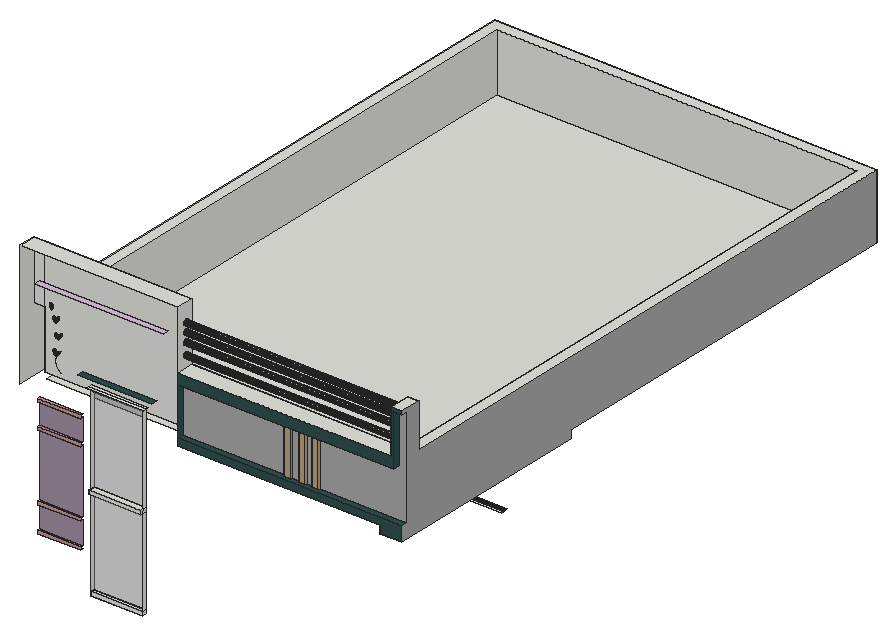
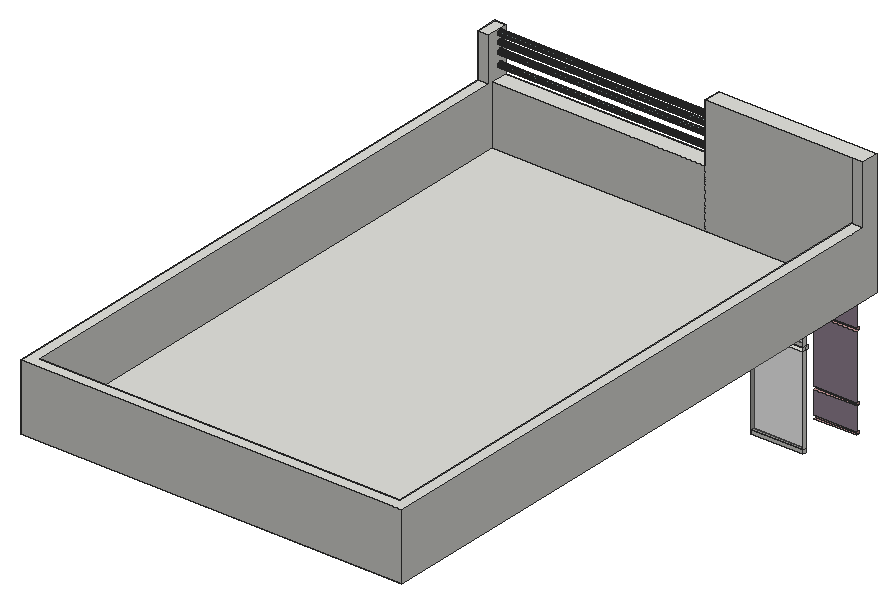
# SketchUp Ruby script. Lengths in inches.
U = 1.inch
M = Sketchup.active_model
def pt(a) = Geom::Point3d.new(a.map { |v| v * U })
def face(e, loops, mat)
  f = e.add_face(loops[0].map { |a| pt(a) })
  loops[1..].each { |l| e.add_face(l.map { |a| pt(a) }).erase! }
  f.material = f.back_material = mat if mat
  f
end
# faces: each face lists its corners as indices into pts; further lists are holes
def faces(e, pts, list, mat = nil) = list.each { |f| face(e, (f[0].is_a?(Array) ? f : [f]).map { |l| l.map { |i| pts[i] } }, mat) }
# xy, xz, yz: faces in a plane at the given z, y or x. An outline is a flat list of corners, or four numbers for a rectangle; further outlines are holes
def ring(l) = l.size == 4 ? [[l[0], l[1]], [l[2], l[1]], [l[2], l[3]], [l[0], l[3]]] : l.each_slice(2).to_a
def flat(e, list, mat, &to3) = list.each { |f| face(e, (f[0].is_a?(Array) ? f : [f]).map { |l| ring(l).map { |u, v| to3.(u, v) } }, mat) }
def xy(e, z, list, mat = nil) = flat(e, list, mat) { |x, y| [x, y, z] }
def xz(e, y, list, mat = nil) = flat(e, list, mat) { |x, z| [x, y, z] }
def yz(e, x, list, mat = nil) = flat(e, list, mat) { |y, z| [x, y, z] }
def lines(e, pts, list) = list.each { |a, b| e.add_line(pt(pts[a]), pt(pts[b])) }
# prism: a flat outline (further loops are holes) pulled along v
def prism(e, loops, v, mat = nil)
  f = face(e, loops, mat); d = Geom::Vector3d.new(v.map { |x| x * U })
  f.pushpull(f.normal.samedirection?(d) ? d.length : -d.length)
end
def box(e, o, s, mat = nil) = prism(e, [[o, [o[0] + s[0], o[1], o[2]], [o[0] + s[0], o[1] + s[1], o[2]], [o[0], o[1] + s[1], o[2]]]], [0, 0, s[2]], mat)
def at(x, y, z, deg = 0) = Geom::Transformation.translation(pt([x, y, z])) * Geom::Transformation.rotation(ORIGIN, Z_AXIS, deg.degrees)
def axes(o, x, y, z) = Geom::Transformation.new([*x, 0, *y, 0, *z, 0, *pt(o).to_a, 1])
def part(name) = M.definitions.add(name)
# library, detail: a bought-in or finely detailed component or shape, given as its bounding box
def library(name, o, s) = part(name).tap { |d| box(d.entities, o, s) }
def detail(e, o, s) = box(e.add_group.entities, o, s)
def put(e, d, t, mat = nil) = e.add_instance(d, t).tap { |i| i.material = mat if mat }
def group(e, t, mat = nil) = e.add_group.tap { |g| g.transformation = t; g.material = mat if mat }.entities
root = M.entities
M.materials.add("[0033_NavajoWhite]").color = [186, 162, 126]
M.materials.add("[0078_DarkSlateGray]").color = [47, 79, 79]
M.materials.add("[0090_LightCyan]").color = [165, 188, 188]
M.materials.add("[0118_Thistle]").color = [160, 142, 160]
M.materials.add("[0118_Thistle]1").color = [216, 191, 216]
M.materials.add("[0119_RosyBrown]").color = [198, 151, 151]
M.materials.add("[0124_Purple]").color = [128, 0, 128]
M.materials.add("[0132_LightGray]").color = [169, 169, 169]
M.materials.add("[0136_Charcoal]").color = [35, 35, 35]
M.materials.add("[Translucent Glass Gray]").color = [128, 128, 128]
M.materials["[Translucent Glass Gray]"].alpha = 0.5
xy(root,362.14,[[104.07,77,146.63,80]])
xy(root,365.14,[[104.07,77,146.63,80]])
xy(root,391.54,[[60,78,94.88,80]],"[0119_RosyBrown]")
xy(root,394.13,[[60,78,94.88,80]],"[0119_RosyBrown]")
xy(root,412.82,[[60,78,94.88,80]],"[0119_RosyBrown]")
xy(root,415.1875,[[60,78,94.88,80]],"[0119_RosyBrown]")
xy(root,418.73,[[210.99,246,254.89,248],[260.89,246,304.8,248]])
xy(root,421.73,[[257.89,248,259.89,250]])
xy(root,421.73,[[207.99,246,257.89,248],[257.89,246,259.89,248],[259.89,246,307.8,248]],"[0136_Charcoal]")
xy(root,437.14,[[104.07,75,146.63,80]])
xy(root,440.14,[[104.07,75,146.63,80]])
xy(root,467.57,[[60,78,94.88,80]],"[0119_RosyBrown]")
xy(root,469.9375,[[60,78,94.88,80]],"[0119_RosyBrown]")
xy(root,488.13,[[60,78,94.88,80]],"[0119_RosyBrown]")
xy(root,490.5,[[60,78,94.88,80]],"[0119_RosyBrown]")
xy(root,492,[[342,75,360,248]],"[0078_DarkSlateGray]")
xy(root,498,[[[177,75,177,91,57,91,57,248,342,248,342,75],[209.97,142.3125,210.74,142.46,211.45,142.79,212.04,143.3,212.49,143.95,212.75,144.68,212.8125,145.46,212.67,146.23,212.33,146.94,211.82,147.54,211.18,147.98,210.44,148.24,209.66,148.3,208.89,148.16,208.18,147.83,207.59,147.32,207.14,146.67,206.88,145.93,206.82,145.15,206.96,144.38,207.3,143.68,207.81,143.08,208.45,142.64,209.19,142.375],[279.78,204.125,280.55,204.27,281.26,204.6,281.86,205.11,282.3,205.76,282.5625,206.5,282.625,207.28,282.48,208.05,282.14,208.75,281.64,209.35,280.99,209.79,280.25,210.06,279.47,210.12,278.7,209.97,277.99,209.64,277.4,209.13,276.95,208.48,276.69,207.75,276.63,206.96,276.77,206.19,277.11,205.49,277.62,204.89,278.26,204.45,279,204.1875],[279.78,142.3125,280.55,142.46,281.26,142.79,281.86,143.3,282.3,143.95,282.5625,144.68,282.625,145.46,282.48,146.23,282.14,146.94,281.64,147.54,280.99,147.98,280.25,148.24,279.47,148.3,278.7,148.16,277.99,147.83,277.4,147.32,276.95,146.67,276.69,145.93,276.63,145.15,276.77,144.38,277.11,143.68,277.62,143.08,278.26,142.64,279,142.375],[209.97,203.6875,210.74,203.83,211.45,204.17,212.04,204.68,212.49,205.32,212.75,206.06,212.8125,206.84,212.67,207.61,212.33,208.32,211.82,208.91,211.18,209.36,210.44,209.62,209.66,209.68,208.89,209.54,208.18,209.2,207.59,208.69,207.14,208.05,206.88,207.31,206.82,206.53,206.96,205.76,207.3,205.05,207.81,204.45,208.45,204.01,209.19,203.75]],[209.97,142.3125,209.19,142.375,208.45,142.64,207.81,143.08,207.3,143.68,206.96,144.38,206.82,145.15,206.88,145.93,207.14,146.67,207.59,147.32,208.18,147.83,208.89,148.16,209.66,148.3,210.44,148.24,211.18,147.98,211.82,147.54,212.33,146.94,212.67,146.23,212.8125,145.46,212.75,144.68,212.49,143.95,212.04,143.3,211.45,142.79,210.74,142.46],[279.78,142.3125,279,142.375,278.26,142.64,277.62,143.08,277.11,143.68,276.77,144.38,276.63,145.15,276.69,145.93,276.95,146.67,277.4,147.32,277.99,147.83,278.7,148.16,279.47,148.3,280.25,148.24,280.99,147.98,281.64,147.54,282.14,146.94,282.48,146.23,282.625,145.46,282.5625,144.68,282.3,143.95,281.86,143.3,281.26,142.79,280.55,142.46],[209.97,203.6875,209.19,203.75,208.45,204.01,207.81,204.45,207.3,205.05,206.96,205.76,206.82,206.53,206.88,207.31,207.14,208.05,207.59,208.69,208.18,209.2,208.89,209.54,209.66,209.68,210.44,209.62,211.18,209.36,211.82,208.91,212.33,208.32,212.67,207.61,212.8125,206.84,212.75,206.06,212.49,205.32,212.04,204.68,211.45,204.17,210.74,203.83],[279.78,204.125,279,204.1875,278.26,204.45,277.62,204.89,277.11,205.49,276.77,206.19,276.63,206.96,276.69,207.75,276.95,208.48,277.4,209.13,277.99,209.64,278.7,209.97,279.47,210.12,280.25,210.06,280.99,209.79,281.64,209.35,282.14,208.75,282.48,208.05,282.625,207.28,282.5625,206.5,282.3,205.76,281.86,205.11,281.26,204.6,280.55,204.27],
  [[48,248,360,560],[186,257,351,551],[57,257,177,551]]])
xy(root,504,[[57,89,351,551]])
xy(root,504,[[177,75,360,75,360,80,288.56,80,288.56,78.5,283.23,78.5,283.23,80,278.12,80,278.12,78.5,272.79,78.5,272.79,80,266.31,80,266.31,78.5,260.98,78.5,260.98,80,177,80]],"[0078_DarkSlateGray]")
xy(root,512.14,[[104.07,77,146.63,80]])
xy(root,514.14,[[102.07,75,148.63,77],[102.07,77,148.63,80]])
xy(root,521.33,[[94.88,75,155.82,80]],"[0078_DarkSlateGray]")
xy(root,543,[[177,75,177,80,260.98,80,260.98,78.5,266.31,78.5,266.31,80,272.79,80,272.79,78.5,278.12,78.5,278.12,80,283.23,80,283.23,78.5,288.56,78.5,288.56,80,353.5,80,353.5,75]],"[0078_DarkSlateGray]")
xy(root,552,[[177,75,351,89],[48,89,57,89,57,551,351,551,351,92,360,92,360,560,48,560]])
xy(root,576,[[60,75,165,80]],"[0118_Thistle]1")
xy(root,585,[[353.5,75,360,80]])
xy(root,588,[[351,75,360,92]])
xy(root,600,[[48,75,177,89]])
xz(root,75,[[104.07,437.14,146.63,440.14]])
xz(root,75,[[342,492,360,492,360,504,177,504,177,498,342,498],[177,543,353.5,543,353.5,585,360,585,360,588,351,588,351,552,177,552]],"[0078_DarkSlateGray]")
xz(root,77,[[104.07,362.14,146.63,365.14]])
xz(root,78,[[60,391.54,94.88,394.13],[60,412.82,94.88,415.1875],[60,467.57,94.88,469.9375],[60,488.13,94.88,490.5]],"[0119_RosyBrown]")
xz(root,78.5,[[260.98,504,266.31,543],[272.79,504,278.12,543],[283.23,504,288.56,543]],"[0033_NavajoWhite]")
xz(root,79,[[73.8,526.12,73.84,526.22,73.93,526.2,73.88,526.35,73.91,526.44,73.83,527.41,73.76,527.67,73.61,528.06,73.43,528.42,73.2,528.77,72.94,529.09,72.65,529.38,72.34,529.64,71.99,529.87,71.63,530.06,71.61,529.65,71.63,529.23,71.7,528.83,71.81,528.43,71.96,528.05,72.14,527.68,72.37,527.34,72.625,527.02,72.91,526.73,73.23,526.47,73.58,526.24],[73.93,526.2,74.32,526.34,74.6875,526.52,75.04,526.73,75.36,526.98,75.66,527.26,75.93,527.57,76.17,527.91,76.37,528.27,76.53,528.65,76.65,529.04,76.73,529.44,76.77,529.85,76.38,529.71,76.01,529.54,75.66,529.32,75.33,529.08,75.03,528.79,74.76,528.48,74.53,528.15,74.41,527.93,73.97,526.61],[75.99,538.9375,75.53,540.22,75.39,540.46,75.15,540.79,74.88,541.1,74.57,541.37,74.24,541.61,73.88,541.82,73.51,541.99,73.12,542.12,72.72,542.21,72.81,541.81,72.9375,541.42,73.1,541.04,73.3125,540.6875,73.55,540.35,73.83,540.05,74.13,539.77,74.47,539.53,74.82,539.32,75.2,539.15,75.59,539.03],[75.99,538.9375,76.31,539.1875,76.61,539.47,76.88,539.78,77.12,540.12,77.32,540.48,77.48,540.86,77.6,541.25,77.68,541.65,77.71,542.0625,77.71,542.47,77.66,542.88,77.57,543.28,77.24,543.03,76.94,542.75,76.68,542.44,76.44,542.1,76.24,541.74,76.08,541.36,75.96,540.97,75.96,540.96],[74.27,550.51,73.82,551.8,73.68,552.03,73.4375,552.37,73.16,552.67,72.86,552.95,72.52,553.19,72.17,553.4,71.79,553.57,71.4,553.69,71,553.78,71.09,553.38,71.22,552.99,71.39,552.62,71.59,552.26,71.84,551.93,72.11,551.625,72.42,551.35,72.75,551.11,73.11,550.9,73.48,550.73,73.87,550.6],
  [74.27,550.51,74.58,550.79,74.85,551.1,75.09,551.43,75.29,551.79,75.46,552.16,75.59,552.55,75.67,552.96,75.72,553.37,75.72,553.78,75.68,554.1875,75.59,554.59,75.47,554.98,75.17,554.7,74.89,554.4,74.65,554.0625,74.45,553.71,74.28,553.33,74.15,552.9375,74.07,552.54,74.02,552.13,74.02,551.72,74.0625,551.31,74.08,551.22,74.18,550.91],[70.59,558.8,70.66,559.21,70.7,559.62,70.7,560.03,70.65,560.43,70.56,560.84,70.43,561.23,70.26,561.6,70.05,561.95,69.81,562.29,69.53,562.59,69.22,562.86,68.89,563.11,68.8125,562.7,68.77,562.29,68.78,561.88,68.83,561.47,68.92,561.07,69.05,560.68,69.22,560.31,69.43,559.95,69.67,559.62,69.95,559.32,70.25,559.04]],"[0124_Purple]")
xz(root,80,[[104.07,362.14,146.63,365.14],[73.86,526.09,73.93,526.2,73.84,526.22,73.8,526.12],[73.93,526.2,73.91,526.44,73.88,526.35],[73.97,526.61,74.41,527.93,74.33,527.79,74.17,527.41,74.05,527.02],[75.99,538.9375,75.96,540.96,75.88,540.57,75.85,540.16,75.85,539.75,75.9,539.34],
  [74.27,550.51,74.15,550.9,74.08,551.22,74.05,551.3,73.88,551.68,73.82,551.8],[74.27,550.51,74.18,550.91,74.08,551.22,74.15,550.9]])
xz(root,80,[[60,394.13,94.88,412.82],[60,415.1875,94.88,467.57],[60,469.9375,94.88,488.13]],"[0118_Thistle]")
xz(root,80,[[177,504,260.98,543],[266.31,504,272.79,543],[278.12,504,283.23,543],[288.56,504,360,504,360,585,353.5,585,353.5,543,288.56,543]],"[0132_LightGray]")
xz(root,80,[[104.07,365.14,146.63,437.14],[104.07,440.14,146.63,512.14]],"[Translucent Glass Gray]")
xz(root,89,[[57,504,177,600],[177,504,351,552],[48,552,57,600]])
xz(root,92,[[351,552,360,588]])
xz(root,248,[[342,492,351,498],[351,492,360,498]])
xz(root,551,[[57,504,351,552]])
xz(root,560,[[48,498,360,552]])
yz(root,48,[[75,498,75,600,89,600,89,552,560,552,560,498]])
yz(root,57,[[89,504,551,552]])
yz(root,70.7,[[79,559.62,80,560.03]],"[0124_Purple]")
yz(root,74.02,[[79,551.72,80,552.13]],"[0124_Purple]")
yz(root,75.72,[[79,553.37,80,553.78]],"[0124_Purple]")
yz(root,75.96,[[79,540.96,80,540.97]],"[0124_Purple]")
yz(root,77.71,[[79,542.0625,80,542.47]],"[0124_Purple]")
yz(root,104.07,[[77,362.14,80,365.14],[77,365.14,80,437.14],[75,437.14,77,440.14],[77,437.14,80,440.14],[77,440.14,80,512.14]])
yz(root,146.63,[[77,362.14,80,365.14],[77,365.14,80,437.14],[75,437.14,77,440.14],[77,437.14,80,440.14],[77,440.14,80,512.14]])
yz(root,177,[[[75,552,89,600],[82,560.12,81.48,560.18,81,560.38,80.59,560.7,80.27,561.12,80.07,561.6,80,562.12,80.07,562.63,80.27,563.12,80.59,563.53,81,563.85,81.48,564.05,82,564.12,82.52,564.05,83,563.85,83.41,563.53,83.73,563.12,83.93,562.63,84,562.12,83.93,561.6,83.73,561.12,83.41,560.7,83,560.38,82.52,560.18],[82,583.68,81.48,583.75,81,583.95,80.59,584.26,80.27,584.68,80.07,585.16,80,585.68,80.07,586.2,80.27,586.68,80.59,587.09,81,587.41,81.48,587.61,82,587.68,82.52,587.61,83,587.41,83.41,587.09,83.73,586.68,83.93,586.2,84,585.68,83.93,585.16,83.73,584.68,83.41,584.26,83,583.95,82.52,583.75],[82,569.55,81.48,569.62,81,569.82,80.59,570.14,80.27,570.55,80.07,571.04,80,571.55,80.07,572.07,80.27,572.55,80.59,572.97,81,573.29,81.48,573.49,82,573.55,82.52,573.49,83,573.29,83.41,572.97,83.73,572.55,83.93,572.07,84,571.55,83.93,571.04,83.73,570.55,83.41,570.14,83,569.82,82.52,569.62],[82,576.8,81.48,576.87,81,577.07,80.59,577.39,80.27,577.8,80.07,578.29,80,578.8,80.07,579.32,80.27,579.8,80.59,580.22,81,580.54,81.48,580.74,82,580.8,82.52,580.74,83,580.54,83.41,580.22,83.73,579.8,83.93,579.32,84,578.8,83.93,578.29,83.73,577.8,83.41,577.39,83,577.07,82.52,576.87]],[82,560.12,81.48,560.18,81,560.38,80.59,560.7,80.27,561.12,80.07,561.6,80,562.12,80.07,562.63,80.27,563.12,80.59,563.53,81,563.85,81.48,564.05,82,564.12,82.52,564.05,83,563.85,83.41,563.53,83.73,563.12,83.93,562.63,84,562.12,83.93,561.6,83.73,561.12,83.41,560.7,83,560.38,82.52,560.18],[82,569.55,81.48,569.62,81,569.82,80.59,570.14,80.27,570.55,80.07,571.04,80,571.55,80.07,572.07,80.27,572.55,80.59,572.97,81,573.29,81.48,573.49,82,573.55,82.52,573.49,83,573.29,83.41,572.97,83.73,572.55,83.93,572.07,84,571.55,83.93,571.04,83.73,570.55,83.41,570.14,83,569.82,82.52,569.62],[82,576.8,81.48,576.87,81,577.07,80.59,577.39,80.27,577.8,80.07,578.29,80,578.8,80.07,579.32,80.27,579.8,80.59,580.22,81,580.54,81.48,580.74,82,580.8,82.52,580.74,83,580.54,83.41,580.22,83.73,579.8,83.93,579.32,84,578.8,83.93,578.29,83.73,577.8,83.41,577.39,83,577.07,82.52,576.87],[82,583.68,81.48,583.75,81,583.95,80.59,584.26,80.27,584.68,80.07,585.16,80,585.68,80.07,586.2,80.27,586.68,80.59,587.09,81,587.41,81.48,587.61,82,587.68,82.52,587.61,83,587.41,83.41,587.09,83.73,586.68,83.93,586.2,84,585.68,83.93,585.16,83.73,584.68,83.41,584.26,83,583.95,82.52,583.75]])
yz(root,177,[[75,504,80,543]],"[0078_DarkSlateGray]")
yz(root,260.98,[[78.5,504,80,543]],"[0033_NavajoWhite]")
yz(root,266.31,[[78.5,504,80,543]],"[0033_NavajoWhite]")
yz(root,272.79,[[78.5,504,80,543]],"[0033_NavajoWhite]")
yz(root,278.12,[[78.5,504,80,543]],"[0033_NavajoWhite]")
yz(root,283.23,[[78.5,504,80,543]],"[0033_NavajoWhite]")
yz(root,288.56,[[78.5,504,80,543]],"[0033_NavajoWhite]")
yz(root,342,[[75,492,248,498]],"[0078_DarkSlateGray]")
yz(root,351,[[[89,504,89,552,75,552,75,588,92,588,92,552,551,552,551,504],[82,583.68,82.52,583.75,83,583.95,83.41,584.26,83.73,584.68,83.93,585.16,84,585.68,83.93,586.2,83.73,586.68,83.41,587.09,83,587.41,82.52,587.61,82,587.68,81.48,587.61,81,587.41,80.59,587.09,80.27,586.68,80.07,586.2,80,585.68,80.07,585.16,80.27,584.68,80.59,584.26,81,583.95,81.48,583.75],[82,560.12,82.52,560.18,83,560.38,83.41,560.7,83.73,561.12,83.93,561.6,84,562.12,83.93,562.63,83.73,563.12,83.41,563.53,83,563.85,82.52,564.05,82,564.12,81.48,564.05,81,563.85,80.59,563.53,80.27,563.12,80.07,562.63,80,562.12,80.07,561.6,80.27,561.12,80.59,560.7,81,560.38,81.48,560.18],[82,569.55,82.52,569.62,83,569.82,83.41,570.14,83.73,570.55,83.93,571.04,84,571.55,83.93,572.07,83.73,572.55,83.41,572.97,83,573.29,82.52,573.49,82,573.55,81.48,573.49,81,573.29,80.59,572.97,80.27,572.55,80.07,572.07,80,571.55,80.07,571.04,80.27,570.55,80.59,570.14,81,569.82,81.48,569.62],[82,576.8,82.52,576.87,83,577.07,83.41,577.39,83.73,577.8,83.93,578.29,84,578.8,83.93,579.32,83.73,579.8,83.41,580.22,83,580.54,82.52,580.74,82,580.8,81.48,580.74,81,580.54,80.59,580.22,80.27,579.8,80.07,579.32,80,578.8,80.07,578.29,80.27,577.8,80.59,577.39,81,577.07,81.48,576.87]]])
yz(root,353.5,[[75,543,80,585]],"[0078_DarkSlateGray]")
yz(root,360,[[75,492,248,492,248,498,560,498,560,552,92,552,92,588,75,588,75,585,80,585,80,504,75,504]],"[0132_LightGray]")
p = [[73.58,80,526.24],[73.8,80,526.12],[73.8,79,526.12],[73.58,79,526.24],[73.84,80,526.22],[73.84,79,526.22],
  [73.23,80,526.47],[73.23,79,526.47],[73.93,80,526.2],[73.93,79,526.2],[73.88,80,526.35],[73.88,79,526.35],
  [73.97,80,526.61],[73.97,79,526.61],[74.32,80,526.34],[74.32,79,526.34],[73.91,80,526.44],[73.91,79,526.44],
  [74.6875,80,526.52],[74.6875,79,526.52],[73.83,80,527.41],[73.83,79,527.41],[72.91,80,526.73],[72.91,79,526.73],
  [75.04,80,526.73],[75.04,79,526.73],[74.41,80,527.93],[74.41,79,527.93],[72.625,80,527.02],[72.625,79,527.02],
  [75.36,80,526.98],[75.36,79,526.98],[72.37,80,527.34],[72.37,79,527.34],[75.66,80,527.26],[75.66,79,527.26],
  [72.14,80,527.68],[72.14,79,527.68],[75.93,80,527.57],[75.93,79,527.57],[73.76,80,527.67],[73.76,79,527.67],
  [76.17,80,527.91],[76.17,79,527.91],[71.96,80,528.05],[71.96,79,528.05],[73.61,80,528.06],[73.61,79,528.06],
  [74.53,80,528.15],[74.53,79,528.15],[76.37,80,528.27],[76.37,79,528.27],[71.81,80,528.43],[71.81,79,528.43],
  [73.43,80,528.42],[73.43,79,528.42],[74.76,80,528.48],[74.76,79,528.48],[76.53,80,528.65],[76.53,79,528.65],
  [71.7,80,528.83],[71.7,79,528.83],[73.2,80,528.77],[73.2,79,528.77],[75.03,80,528.79],[75.03,79,528.79],
  [76.65,80,529.04],[76.65,79,529.04],[71.63,80,529.23],[71.63,79,529.23],[72.94,80,529.09],[72.94,79,529.09],
  [75.33,80,529.08],[75.33,79,529.08],[76.73,80,529.44],[76.73,79,529.44],[72.65,80,529.38],[72.65,79,529.38],
  [75.66,80,529.32],[75.66,79,529.32],[71.61,80,529.65],[71.61,79,529.65],[76.01,80,529.54],[76.01,79,529.54],
  [72.34,80,529.64],[72.34,79,529.64],[76.77,80,529.85],[76.77,79,529.85],[76.38,80,529.71],[76.38,79,529.71],
  [71.63,80,530.06],[71.63,79,530.06],[71.99,80,529.87],[71.99,79,529.87],[75.99,80,538.9375],[75.53,80,540.22],
  [75.53,79,540.22],[75.99,79,538.9375],[75.59,80,539.03],[75.59,79,539.03],[75.96,80,540.96],[75.96,79,540.96],
  [76.31,80,539.1875],[76.31,79,539.1875],[75.2,80,539.15],[75.2,79,539.15],[74.82,80,539.32],[74.82,79,539.32],
  [76.61,80,539.47],[76.61,79,539.47],[74.47,80,539.53],[74.47,79,539.53],[74.13,80,539.77],[74.13,79,539.77],
  [76.88,80,539.78],[76.88,79,539.78],[73.83,80,540.05],[73.83,79,540.05],[77.12,80,540.12],[77.12,79,540.12],
  [73.55,80,540.35],[73.55,79,540.35],[77.32,80,540.48],[77.32,79,540.48],[75.39,80,540.46],[75.39,79,540.46],
  [73.3125,80,540.6875],[73.3125,79,540.6875],[75.15,80,540.79],[75.15,79,540.79],[77.48,80,540.86],[77.48,79,540.86],
  [73.1,80,541.04],[73.1,79,541.04],[74.88,80,541.1],[74.88,79,541.1],[77.6,80,541.25],[77.6,79,541.25],
  [72.9375,80,541.42],[72.9375,79,541.42],[76.08,80,541.36],[75.96,80,540.97],[75.96,79,540.97],[76.08,79,541.36],
  [74.57,80,541.37],[74.57,79,541.37],[77.68,80,541.65],[77.68,79,541.65],[72.81,80,541.81],[72.81,79,541.81],
  [74.24,80,541.61],[74.24,79,541.61],[76.24,80,541.74],[76.24,79,541.74],[73.88,80,541.82],[73.88,79,541.82],
  [76.44,80,542.1],[76.44,79,542.1],[77.71,80,542.0625],[77.71,79,542.0625],[72.72,80,542.21],[72.72,79,542.21],
  [73.51,80,541.99],[73.51,79,541.99],[73.12,80,542.12],[73.12,79,542.12],[76.68,80,542.44],[76.68,79,542.44],
  [76.94,80,542.75],[76.94,79,542.75],[77.71,80,542.47],[77.66,80,542.88],[77.66,79,542.88],[77.71,79,542.47],
  [77.24,80,543.03],[77.24,79,543.03],[77.57,80,543.28],[77.57,79,543.28],[74.27,80,550.51],[73.82,80,551.8],
  [73.82,79,551.8],[74.27,79,550.51],[73.87,80,550.6],[73.87,79,550.6],[74.18,80,550.91],[74.18,79,550.91],
  [74.58,80,550.79],[74.58,79,550.79],[73.48,80,550.73],[73.48,79,550.73],[73.11,80,550.9],[73.11,79,550.9],
  [74.85,80,551.1],[74.85,79,551.1],[72.75,80,551.11],[72.75,79,551.11],[74.08,80,551.22],[74.08,79,551.22],
  [72.42,80,551.35],[72.42,79,551.35],[75.09,80,551.43],[75.09,79,551.43],[74.0625,80,551.31],[74.0625,79,551.31],
  [72.11,80,551.625],[72.11,79,551.625],[74.02,80,551.72],[74.02,79,551.72],[75.29,80,551.79],[75.29,79,551.79],
  [71.84,80,551.93],[71.84,79,551.93],[73.68,80,552.03],[73.68,79,552.03],[75.46,80,552.16],[75.46,79,552.16],
  [71.59,80,552.26],[71.59,79,552.26],[73.4375,80,552.37],[73.4375,79,552.37],[74.07,80,552.54],[74.02,80,552.13],
  [74.02,79,552.13],[74.07,79,552.54],[75.59,80,552.55],[75.59,79,552.55],[71.39,80,552.62],[71.39,79,552.62],
  [73.16,80,552.67],[73.16,79,552.67],[74.15,80,552.9375],[74.15,79,552.9375],[71.22,80,552.99],[71.22,79,552.99],
  [75.67,80,552.96],[75.67,79,552.96],[72.86,80,552.95],[72.86,79,552.95],[72.52,80,553.19],[72.52,79,553.19],
  [74.28,80,553.33],[74.28,79,553.33],[71.09,80,553.38],[71.09,79,553.38],[75.72,80,553.37],[75.72,79,553.37],
  [72.17,80,553.4],[72.17,79,553.4],[74.45,80,553.71],[74.45,79,553.71],[71,80,553.78],[71,79,553.78],
  [71.79,80,553.57],[71.79,79,553.57],[71.4,80,553.69],[71.4,79,553.69],[74.65,80,554.0625],[74.65,79,554.0625],
  [75.72,80,553.78],[75.68,80,554.1875],[75.68,79,554.1875],[75.72,79,553.78],[74.89,80,554.4],[74.89,79,554.4],
  [75.59,80,554.59],[75.59,79,554.59],[75.17,80,554.7],[75.17,79,554.7],[75.47,80,554.98],[75.47,79,554.98],
  [70.25,80,559.04],[70.59,80,558.8],[70.59,79,558.8],[70.25,79,559.04],[70.66,80,559.21],[70.66,79,559.21],
  [69.95,80,559.32],[69.95,79,559.32],[70.7,80,559.62],[70.7,79,559.62],[69.67,80,559.62],[69.67,79,559.62],
  [69.43,80,559.95],[69.43,79,559.95],[69.22,80,560.31],[69.22,79,560.31],[70.7,80,560.03],[70.65,80,560.43],
  [70.65,79,560.43],[70.7,79,560.03],[177,81.48,560.18],[177,82,560.12],[351,82,560.12],[351,81.48,560.18],
  [177,82.52,560.18],[351,82.52,560.18],[177,81,560.38],[351,81,560.38],[177,83,560.38],[351,83,560.38],
  [69.05,80,560.68],[69.05,79,560.68],[70.56,80,560.84],[70.56,79,560.84],[177,80.59,560.7],[351,80.59,560.7],
  [177,83.41,560.7],[351,83.41,560.7],[68.92,80,561.07],[68.92,79,561.07],[177,80.27,561.12],[351,80.27,561.12],
  [177,83.73,561.12],[351,83.73,561.12],[70.43,80,561.23],[70.43,79,561.23],[68.83,80,561.47],[68.83,79,561.47],
  [177,80.07,561.6],[351,80.07,561.6],[177,83.93,561.6],[351,83.93,561.6],[70.26,80,561.6],[70.26,79,561.6],
  [68.78,80,561.88],[68.78,79,561.88],[70.05,80,561.95],[70.05,79,561.95],[177,80,562.12],[351,80,562.12],
  [177,84,562.12],[351,84,562.12],[68.77,80,562.29],[68.77,79,562.29],[69.81,80,562.29],[69.81,79,562.29],
  [177,80.07,562.63],[351,80.07,562.63],[177,83.93,562.63],[351,83.93,562.63],[68.8125,80,562.7],[68.8125,79,562.7],
  [69.53,80,562.59],[69.53,79,562.59],[69.22,80,562.86],[69.22,79,562.86],[177,80.27,563.12],[351,80.27,563.12],
  [177,83.73,563.12],[351,83.73,563.12],[68.89,80,563.11],[68.89,79,563.11],[177,80.59,563.53],[351,80.59,563.53],
  [177,83.41,563.53],[351,83.41,563.53],[177,81,563.85],[351,81,563.85],[177,83,563.85],[351,83,563.85],
  [177,81.48,564.05],[351,81.48,564.05],[177,82.52,564.05],[351,82.52,564.05],[177,82,564.12],[351,82,564.12],
  [177,81,569.82],[177,81.48,569.62],[351,81.48,569.62],[351,81,569.82],[177,82,569.55],[351,82,569.55],
  [177,82.52,569.62],[351,82.52,569.62],[177,83,569.82],[351,83,569.82],[177,80.59,570.14],[351,80.59,570.14],
  [177,83.41,570.14],[351,83.41,570.14],[177,80.27,570.55],[351,80.27,570.55],[177,83.73,570.55],[351,83.73,570.55],
  [177,80.07,571.04],[351,80.07,571.04],[177,83.93,571.04],[351,83.93,571.04],[177,80,571.55],[351,80,571.55],
  [177,84,571.55],[351,84,571.55],[177,80.07,572.07],[351,80.07,572.07],[177,83.93,572.07],[351,83.93,572.07],
  [177,80.27,572.55],[351,80.27,572.55],[177,83.73,572.55],[351,83.73,572.55],[177,80.59,572.97],[351,80.59,572.97],
  [177,83.41,572.97],[351,83.41,572.97],[177,81,573.29],[351,81,573.29],[177,83,573.29],[351,83,573.29],
  [177,81.48,573.49],[351,81.48,573.49],[177,82.52,573.49],[351,82.52,573.49],[177,82,573.55],[351,82,573.55],
  [177,81.48,576.87],[177,82,576.8],[351,82,576.8],[351,81.48,576.87],[177,82.52,576.87],[351,82.52,576.87],
  [177,81,577.07],[351,81,577.07],[177,83,577.07],[351,83,577.07],[177,80.59,577.39],[351,80.59,577.39],
  [177,83.41,577.39],[351,83.41,577.39],[177,80.27,577.8],[351,80.27,577.8],[177,83.73,577.8],[351,83.73,577.8],
  [177,80.07,578.29],[351,80.07,578.29],[177,83.93,578.29],[351,83.93,578.29],[177,80,578.8],[351,80,578.8],
  [177,84,578.8],[351,84,578.8],[177,80.07,579.32],[351,80.07,579.32],[177,83.93,579.32],[351,83.93,579.32],
  [177,80.27,579.8],[351,80.27,579.8],[177,83.73,579.8],[351,83.73,579.8],[177,80.59,580.22],[351,80.59,580.22],
  [177,83.41,580.22],[351,83.41,580.22],[177,81,580.54],[351,81,580.54],[177,83,580.54],[351,83,580.54],
  [177,81.48,580.74],[351,81.48,580.74],[177,82.52,580.74],[351,82.52,580.74],[177,82,580.8],[351,82,580.8],
  [177,81,583.95],[177,81.48,583.75],[351,81.48,583.75],[351,81,583.95],[177,82,583.68],[351,82,583.68],
  [177,82.52,583.75],[351,82.52,583.75],[177,83,583.95],[351,83,583.95],[177,80.59,584.26],[351,80.59,584.26],
  [177,83.41,584.26],[351,83.41,584.26],[177,80.27,584.68],[351,80.27,584.68],[177,83.73,584.68],[351,83.73,584.68],
  [177,80.07,585.16],[351,80.07,585.16],[177,83.93,585.16],[351,83.93,585.16],[177,80,585.68],[351,80,585.68],
  [177,84,585.68],[351,84,585.68],[177,80.07,586.2],[351,80.07,586.2],[177,83.93,586.2],[351,83.93,586.2],
  [177,80.27,586.68],[351,80.27,586.68],[177,83.73,586.68],[351,83.73,586.68],[177,80.59,587.09],[351,80.59,587.09],
  [177,83.41,587.09],[351,83.41,587.09],[177,81,587.41],[351,81,587.41],[177,83,587.41],[351,83,587.41],
  [177,81.48,587.61],[351,81.48,587.61],[177,82.52,587.61],[351,82.52,587.61],[177,82,587.68],[351,82,587.68],
  [177,82,562.12],[351,82,562.12],[177,82,571.55],[351,82,571.55],[177,82,578.8],[351,82,578.8],
  [177,82,585.68],[351,82,585.68],[73.44,80,525.05],[73.12,80,524.02],[72.92,80,522.96],[72.84,80,521.875],
  [72.9,80,520.79],[73.08,80,519.72],[73.39,80,518.68],[73.81,80,517.69],[74.36,80,516.75],[75.01,80,515.89],
  [75.76,80,515.1],[76.6,80,514.41],[77.51,80,513.83]]
faces(root,p,[[0,1,2,3],[6,0,3,7],[8,14,15,9],[14,18,19,15],[22,6,7,23],[18,24,25,19],[26,12,13,27],[28,22,23,29],
  [24,30,31,25],[32,28,29,33],[30,34,35,31],[36,32,33,37],[34,38,39,35],[20,40,41,21],[38,42,43,39],[44,36,37,45],
  [40,46,47,41],[48,26,27,49],[42,50,51,43],[52,44,45,53],[46,54,55,47],[56,48,49,57],[50,58,59,51],[60,52,53,61],
  [54,62,63,55],[64,56,57,65],[58,66,67,59],[68,60,61,69],[62,70,71,63],[72,64,65,73],[66,74,75,67],[70,76,77,71],
  [78,72,73,79],[80,68,69,81],[82,78,79,83],[76,84,85,77],[74,86,87,75],[88,82,83,89],[90,80,81,91],[84,92,93,85],
  [86,88,89,87],[92,90,91,93],[98,94,97,99],[100,94,97,101],[94,102,103,97],[104,98,99,105],[106,104,105,107],[102,108,109,103],
  [110,106,107,111],[112,110,111,113],[108,114,115,109],[116,112,113,117],[114,118,119,115],[120,116,117,121],[118,122,123,119],[95,124,125,96],
  [126,120,121,127],[124,128,129,125],[122,130,131,123],[132,126,127,133],[128,134,135,129],[130,136,137,131],[138,132,133,139],[140,141,142,143],
  [134,144,145,135],[136,146,147,137],[148,138,139,149],[144,150,151,145],[152,140,143,153],[150,154,155,151],[156,152,153,157],[146,158,159,147],
  [160,148,149,161],[154,162,163,155],[162,164,165,163],[164,160,161,165],[166,156,157,167],[168,166,167,169],[170,171,172,173],[174,168,169,175],
  [171,176,177,172],[176,174,175,177],[182,178,181,183],[178,186,187,181],[188,182,183,189],[190,188,189,191],[186,192,193,187],[194,190,191,195],
  [198,194,195,199],[192,200,201,193],[202,196,197,203],[204,198,199,205],[206,202,203,207],[200,208,209,201],[210,204,205,211],[179,212,213,180],
  [208,214,215,209],[216,210,211,217],[212,218,219,213],[220,221,222,223],[214,224,225,215],[226,216,217,227],[218,228,229,219],[230,220,223,231],
  [232,226,227,233],[224,234,235,225],[228,236,237,229],[236,238,239,237],[240,230,231,241],[242,232,233,243],[234,244,245,235],[238,246,247,239],
  [248,240,241,249],[250,242,243,251],[246,252,253,247],[252,254,255,253],[254,250,251,255],[256,248,249,257],[258,259,260,261],[262,256,257,263],
  [259,264,265,260],[266,262,263,267],[264,268,269,265],[268,266,267,269],[270,271,272,273],[271,274,275,272],[276,270,273,277],[274,278,279,275],
  [280,276,277,281],[282,280,281,283],[284,282,283,285],[286,287,288,289],[300,284,285,301],[287,302,303,288],[308,300,301,309],[302,314,315,303],
  [316,308,309,317],[314,322,323,315],[324,316,317,325],[322,326,327,323],[332,324,325,333],[326,334,335,327],[340,332,333,341],[334,342,343,335],
  [342,344,345,343],[350,340,341,351],[344,350,351,345]],"[0124_Purple]")
faces(root,p,[[1,4,5,2],[4,8,9,5],[8,10,11,9],[12,8,9,13],[10,16,17,11],[16,20,21,17],[94,95,96,97],[178,179,180,181],
  [184,178,181,185],[196,184,185,197]])
faces(root,p,[[290,291,292,293],[291,294,295,292],[296,290,293,297],[294,298,299,295],[304,296,297,305],[298,306,307,299],[310,304,305,311],[306,312,313,307],
  [318,310,311,319],[312,320,321,313],[328,318,319,329],[320,330,331,321],[336,328,329,337],[330,338,339,331],[346,336,337,347],[338,348,349,339],
  [352,346,347,353],[348,354,355,349],[356,352,353,357],[354,358,359,355],[360,356,357,361],[358,362,363,359],[364,360,361,365],[362,364,365,363],
  [366,367,368,369],[367,370,371,368],[370,372,373,371],[372,374,375,373],[376,366,369,377],[374,378,379,375],[380,376,377,381],[378,382,383,379],
  [384,380,381,385],[382,386,387,383],[388,384,385,389],[386,390,391,387],[392,388,389,393],[390,394,395,391],[396,392,393,397],[394,398,399,395],
  [400,396,397,401],[398,402,403,399],[404,400,401,405],[402,406,407,403],[408,404,405,409],[406,410,411,407],[412,408,409,413],[410,412,413,411],
  [414,415,416,417],[415,418,419,416],[420,414,417,421],[418,422,423,419],[424,420,421,425],[422,426,427,423],[428,424,425,429],[426,430,431,427],
  [432,428,429,433],[430,434,435,431],[436,432,433,437],[434,438,439,435],[440,436,437,441],[438,442,443,439],[444,440,441,445],[442,446,447,443],
  [448,444,445,449],[446,450,451,447],[452,448,449,453],[450,454,455,451],[456,452,453,457],[454,458,459,455],[460,456,457,461],[458,460,461,459],
  [462,463,464,465],[463,466,467,464],[466,468,469,467],[468,470,471,469],[472,462,465,473],[470,474,475,471],[476,472,473,477],[474,478,479,475],
  [480,476,477,481],[478,482,483,479],[484,480,481,485],[482,486,487,483],[488,484,485,489],[486,490,491,487],[492,488,489,493],[490,494,495,491],
  [496,492,493,497],[494,498,499,495],[500,496,497,501],[498,502,503,499],[504,500,501,505],[502,506,507,503],[508,504,505,509],[506,508,509,507]],"[0090_LightCyan]")
lines(root,p,[[510,511],[512,513],[514,515],[516,517],[518,519],[519,520],[520,521],[521,522],[522,523],[523,524],[524,525],[525,526],
  [526,527],[527,528],[528,529],[529,530],[1,518]])
